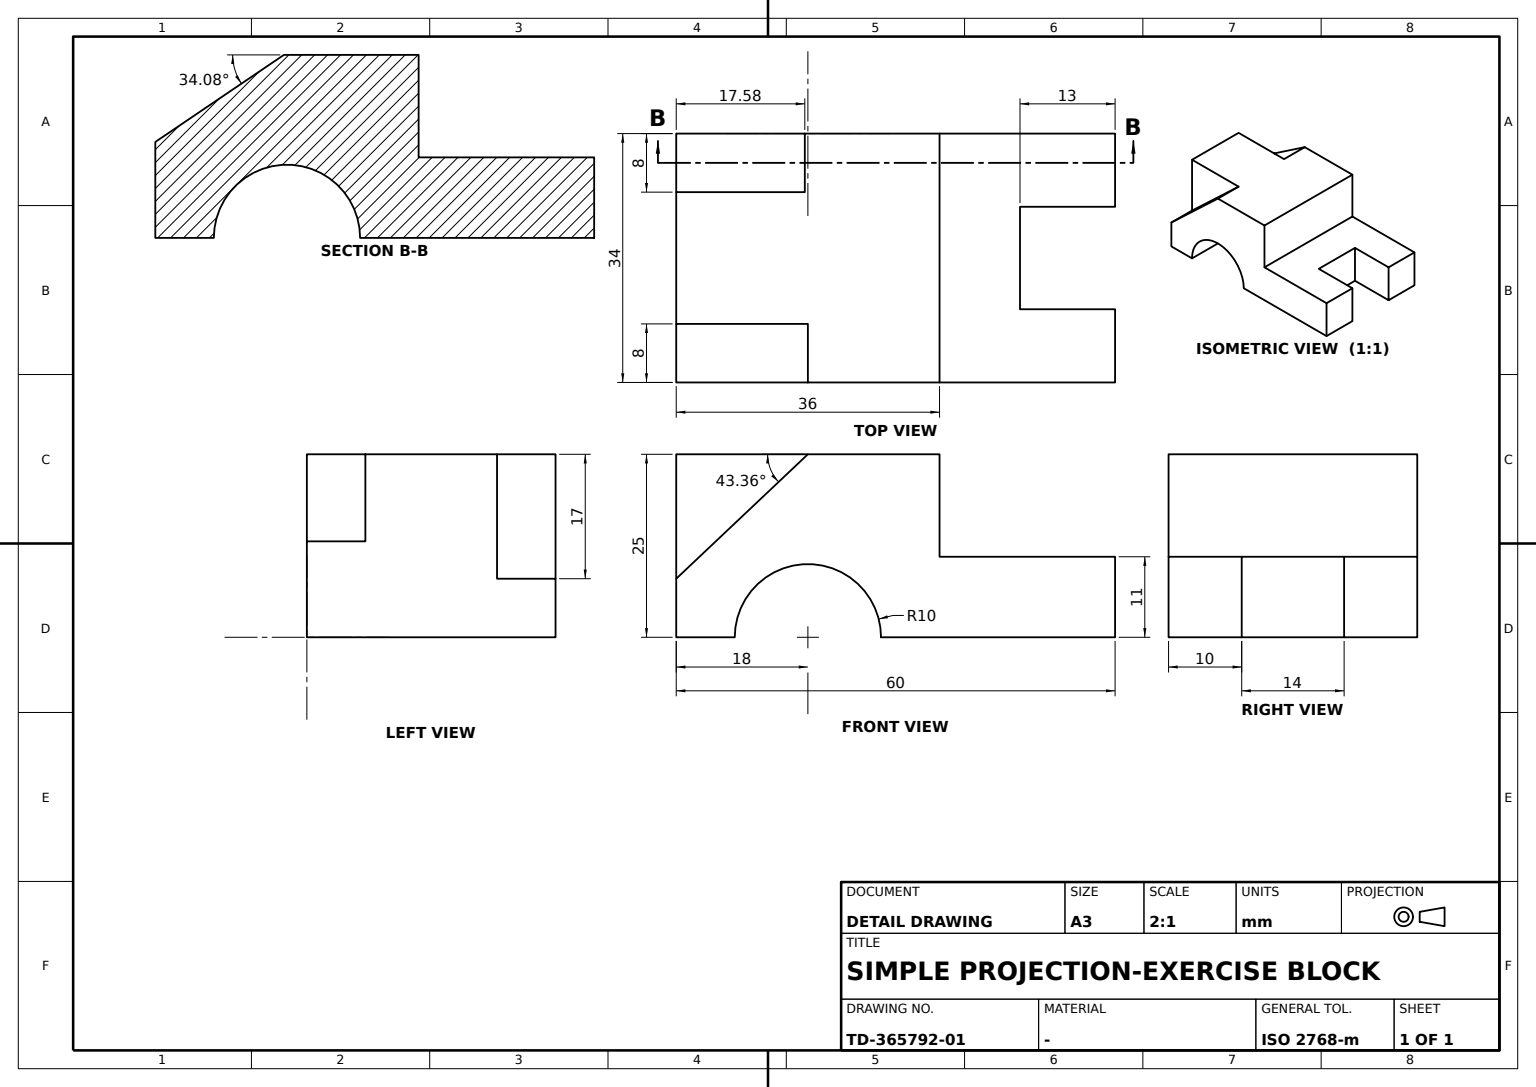
ISO-10303-21;
HEADER;
FILE_DESCRIPTION((''),'2;1');
FILE_NAME('','',(''),(''),'','','');
FILE_SCHEMA(('AUTOMOTIVE_DESIGN'));
ENDSEC;
DATA;
#1=APPLICATION_CONTEXT('');
#2=PRODUCT_CONTEXT('',#1,'mechanical');
#3=PRODUCT('','','',(#2));
#4=PRODUCT_DEFINITION_FORMATION('','',#3);
#5=PRODUCT_DEFINITION_CONTEXT('',#1,'design');
#6=PRODUCT_DEFINITION('','',#4,#5);
#7=PRODUCT_DEFINITION_SHAPE('','',#6);
#8=(LENGTH_UNIT()NAMED_UNIT(*)SI_UNIT(.MILLI.,.METRE.));
#9=(NAMED_UNIT(*)PLANE_ANGLE_UNIT()SI_UNIT($,.RADIAN.));
#10=(NAMED_UNIT(*)SI_UNIT($,.STERADIAN.)SOLID_ANGLE_UNIT());
#11=UNCERTAINTY_MEASURE_WITH_UNIT(LENGTH_MEASURE(0.005),#8,'distance_accuracy_value','');
#12=(GEOMETRIC_REPRESENTATION_CONTEXT(3)GLOBAL_UNCERTAINTY_ASSIGNED_CONTEXT((#11))GLOBAL_UNIT_ASSIGNED_CONTEXT((#8,#9,#10))REPRESENTATION_CONTEXT('',''));
#13=CARTESIAN_POINT('',(-17.,-18.,13.105238));
#14=VERTEX_POINT('',#13);
#15=CARTESIAN_POINT('',(-9.,-18.,13.105238));
#16=VERTEX_POINT('',#15);
#17=DIRECTION('',(1.,0.,0.));
#18=VECTOR('',#17,1000.);
#19=LINE('',#13,#18);
#20=EDGE_CURVE('',#14,#16,#19,.T.);
#21=ORIENTED_EDGE('',*,*,#20,.T.);
#22=CARTESIAN_POINT('',(-9.,-0.420078,25.));
#23=VERTEX_POINT('',#22);
#24=DIRECTION('',(0.,-0.82822958,-0.560388939));
#25=VECTOR('',#24,1000.);
#26=LINE('',#22,#25);
#27=EDGE_CURVE('',#23,#16,#26,.T.);
#28=ORIENTED_EDGE('',*,*,#27,.F.);
#29=CARTESIAN_POINT('',(-17.,-0.420078,25.));
#30=VERTEX_POINT('',#29);
#31=CARTESIAN_POINT('',(0.,-0.420078,25.));
#32=LINE('',#31,#18);
#33=EDGE_CURVE('',#30,#23,#32,.T.);
#34=ORIENTED_EDGE('',*,*,#33,.F.);
#35=CARTESIAN_POINT('',(-17.,-11.735187,17.344077));
#36=LINE('',#35,#25);
#37=EDGE_CURVE('',#30,#14,#36,.T.);
#38=ORIENTED_EDGE('',*,*,#37,.T.);
#39=EDGE_LOOP('',(#21,#28,#34,#38));
#40=FACE_BOUND('',#39,.T.);
#41=DIRECTION('',(0.,-0.560388939,0.82822958));
#42=AXIS2_PLACEMENT_3D('',#29,#41,#24);
#43=PLANE('',#42);
#44=ADVANCED_FACE('',(#40),#43,.T.);
#45=CARTESIAN_POINT('',(-17.,42.,11.));
#46=VERTEX_POINT('',#45);
#47=CARTESIAN_POINT('',(-7.,42.,11.));
#48=VERTEX_POINT('',#47);
#49=CARTESIAN_POINT('',(0.,42.,11.));
#50=LINE('',#49,#18);
#51=EDGE_CURVE('',#46,#48,#50,.T.);
#52=ORIENTED_EDGE('',*,*,#51,.F.);
#53=CARTESIAN_POINT('',(-17.,18.,11.));
#54=VERTEX_POINT('',#53);
#55=CARTESIAN_POINT('',(-17.,0.,11.));
#56=DIRECTION('',(0.,-1.,0.));
#57=VECTOR('',#56,1000.);
#58=LINE('',#55,#57);
#59=EDGE_CURVE('',#46,#54,#58,.T.);
#60=ORIENTED_EDGE('',*,*,#59,.T.);
#61=CARTESIAN_POINT('',(17.,18.,11.));
#62=VERTEX_POINT('',#61);
#63=CARTESIAN_POINT('',(0.,18.,11.));
#64=LINE('',#63,#18);
#65=EDGE_CURVE('',#54,#62,#64,.T.);
#66=ORIENTED_EDGE('',*,*,#65,.T.);
#67=CARTESIAN_POINT('',(17.,42.,11.));
#68=VERTEX_POINT('',#67);
#69=CARTESIAN_POINT('',(17.,0.,11.));
#70=LINE('',#69,#57);
#71=EDGE_CURVE('',#68,#62,#70,.T.);
#72=ORIENTED_EDGE('',*,*,#71,.F.);
#73=CARTESIAN_POINT('',(7.,42.,11.));
#74=VERTEX_POINT('',#73);
#75=EDGE_CURVE('',#74,#68,#50,.T.);
#76=ORIENTED_EDGE('',*,*,#75,.F.);
#77=CARTESIAN_POINT('',(7.,29.,11.));
#78=VERTEX_POINT('',#77);
#79=LINE('',#73,#57);
#80=EDGE_CURVE('',#74,#78,#79,.T.);
#81=ORIENTED_EDGE('',*,*,#80,.T.);
#82=CARTESIAN_POINT('',(-7.,29.,11.));
#83=VERTEX_POINT('',#82);
#84=DIRECTION('',(-1.,0.,0.));
#85=VECTOR('',#84,1000.);
#86=LINE('',#77,#85);
#87=EDGE_CURVE('',#78,#83,#86,.T.);
#88=ORIENTED_EDGE('',*,*,#87,.T.);
#89=DIRECTION('',(0.,1.,0.));
#90=VECTOR('',#89,1000.);
#91=LINE('',#82,#90);
#92=EDGE_CURVE('',#83,#48,#91,.T.);
#93=ORIENTED_EDGE('',*,*,#92,.T.);
#94=EDGE_LOOP('',(#52,#60,#66,#72,#76,#81,#88,#93));
#95=FACE_BOUND('',#94,.T.);
#96=DIRECTION('',(0.,0.,1.));
#97=AXIS2_PLACEMENT_3D('',#49,#96,#56);
#98=PLANE('',#97);
#99=ADVANCED_FACE('',(#95),#98,.T.);
#100=ORIENTED_EDGE('',*,*,#33,.T.);
#101=CARTESIAN_POINT('',(-9.,-18.,25.));
#102=VERTEX_POINT('',#101);
#103=CARTESIAN_POINT('',(-9.,18.,25.));
#104=LINE('',#103,#57);
#105=EDGE_CURVE('',#23,#102,#104,.T.);
#106=ORIENTED_EDGE('',*,*,#105,.T.);
#107=CARTESIAN_POINT('',(9.,-18.,25.));
#108=VERTEX_POINT('',#107);
#109=CARTESIAN_POINT('',(0.,-18.,25.));
#110=LINE('',#109,#18);
#111=EDGE_CURVE('',#102,#108,#110,.T.);
#112=ORIENTED_EDGE('',*,*,#111,.T.);
#113=CARTESIAN_POINT('',(9.,0.,25.));
#114=VERTEX_POINT('',#113);
#115=LINE('',#113,#57);
#116=EDGE_CURVE('',#114,#108,#115,.T.);
#117=ORIENTED_EDGE('',*,*,#116,.F.);
#118=CARTESIAN_POINT('',(17.,0.,25.));
#119=VERTEX_POINT('',#118);
#120=LINE('',#118,#85);
#121=EDGE_CURVE('',#119,#114,#120,.T.);
#122=ORIENTED_EDGE('',*,*,#121,.F.);
#123=CARTESIAN_POINT('',(17.,18.,25.));
#124=VERTEX_POINT('',#123);
#125=LINE('',#118,#57);
#126=EDGE_CURVE('',#124,#119,#125,.T.);
#127=ORIENTED_EDGE('',*,*,#126,.F.);
#128=CARTESIAN_POINT('',(-17.,18.,25.));
#129=VERTEX_POINT('',#128);
#130=CARTESIAN_POINT('',(0.,18.,25.));
#131=LINE('',#130,#18);
#132=EDGE_CURVE('',#129,#124,#131,.T.);
#133=ORIENTED_EDGE('',*,*,#132,.F.);
#134=CARTESIAN_POINT('',(-17.,0.,25.));
#135=LINE('',#134,#57);
#136=EDGE_CURVE('',#129,#30,#135,.T.);
#137=ORIENTED_EDGE('',*,*,#136,.T.);
#138=EDGE_LOOP('',(#100,#106,#112,#117,#122,#127,#133,#137));
#139=FACE_BOUND('',#138,.T.);
#140=AXIS2_PLACEMENT_3D('',#130,#96,#56);
#141=PLANE('',#140);
#142=ADVANCED_FACE('',(#139),#141,.T.);
#143=CARTESIAN_POINT('',(17.,-18.,0.));
#144=VERTEX_POINT('',#143);
#145=CARTESIAN_POINT('',(17.,-10.,0.));
#146=VERTEX_POINT('',#145);
#147=CARTESIAN_POINT('',(17.,0.,0.));
#148=LINE('',#147,#90);
#149=EDGE_CURVE('',#144,#146,#148,.T.);
#150=ORIENTED_EDGE('',*,*,#149,.F.);
#151=CARTESIAN_POINT('',(-17.,-18.,0.));
#152=VERTEX_POINT('',#151);
#153=CARTESIAN_POINT('',(0.,-18.,0.));
#154=LINE('',#153,#18);
#155=EDGE_CURVE('',#152,#144,#154,.T.);
#156=ORIENTED_EDGE('',*,*,#155,.F.);
#157=CARTESIAN_POINT('',(-17.,-10.,0.));
#158=VERTEX_POINT('',#157);
#159=CARTESIAN_POINT('',(-17.,0.,0.));
#160=LINE('',#159,#90);
#161=EDGE_CURVE('',#152,#158,#160,.T.);
#162=ORIENTED_EDGE('',*,*,#161,.T.);
#163=LINE('',#157,#18);
#164=EDGE_CURVE('',#158,#146,#163,.T.);
#165=ORIENTED_EDGE('',*,*,#164,.T.);
#166=EDGE_LOOP('',(#150,#156,#162,#165));
#167=FACE_BOUND('',#166,.T.);
#168=DIRECTION('',(0.,0.,-1.));
#169=AXIS2_PLACEMENT_3D('',#153,#168,#89);
#170=PLANE('',#169);
#171=ADVANCED_FACE('',(#167),#170,.T.);
#172=CARTESIAN_POINT('',(7.,29.,0.));
#173=VERTEX_POINT('',#172);
#174=VECTOR('',#168,1000.);
#175=LINE('',#77,#174);
#176=EDGE_CURVE('',#78,#173,#175,.T.);
#177=ORIENTED_EDGE('',*,*,#176,.F.);
#178=ORIENTED_EDGE('',*,*,#80,.F.);
#179=CARTESIAN_POINT('',(7.,42.,0.));
#180=VERTEX_POINT('',#179);
#181=LINE('',#179,#174);
#182=EDGE_CURVE('',#74,#180,#181,.T.);
#183=ORIENTED_EDGE('',*,*,#182,.T.);
#184=CARTESIAN_POINT('',(7.,-18.,0.));
#185=LINE('',#184,#57);
#186=EDGE_CURVE('',#180,#173,#185,.T.);
#187=ORIENTED_EDGE('',*,*,#186,.T.);
#188=EDGE_LOOP('',(#177,#178,#183,#187));
#189=FACE_BOUND('',#188,.T.);
#190=AXIS2_PLACEMENT_3D('',#73,#17,#56);
#191=PLANE('',#190);
#192=ADVANCED_FACE('',(#189),#191,.F.);
#193=CARTESIAN_POINT('',(17.,-18.,8.));
#194=VERTEX_POINT('',#193);
#195=DIRECTION('',(0.,0.727013153,0.686623533));
#196=VECTOR('',#195,1000.);
#197=LINE('',#193,#196);
#198=EDGE_CURVE('',#194,#119,#197,.T.);
#199=ORIENTED_EDGE('',*,*,#198,.T.);
#200=ORIENTED_EDGE('',*,*,#121,.T.);
#201=CARTESIAN_POINT('',(9.,-18.,8.));
#202=VERTEX_POINT('',#201);
#203=LINE('',#201,#196);
#204=EDGE_CURVE('',#202,#114,#203,.T.);
#205=ORIENTED_EDGE('',*,*,#204,.F.);
#206=CARTESIAN_POINT('',(0.,-18.,8.));
#207=LINE('',#206,#85);
#208=EDGE_CURVE('',#194,#202,#207,.T.);
#209=ORIENTED_EDGE('',*,*,#208,.F.);
#210=EDGE_LOOP('',(#199,#200,#205,#209));
#211=FACE_BOUND('',#210,.T.);
#212=DIRECTION('',(0.,-0.686623533,0.727013153));
#213=AXIS2_PLACEMENT_3D('',#193,#212,#195);
#214=PLANE('',#213);
#215=ADVANCED_FACE('',(#211),#214,.T.);
#216=LINE('',#101,#174);
#217=EDGE_CURVE('',#102,#16,#216,.T.);
#218=ORIENTED_EDGE('',*,*,#217,.F.);
#219=ORIENTED_EDGE('',*,*,#105,.F.);
#220=ORIENTED_EDGE('',*,*,#27,.T.);
#221=EDGE_LOOP('',(#218,#219,#220));
#222=FACE_BOUND('',#221,.T.);
#223=CARTESIAN_POINT('',(-9.,0.,0.));
#224=AXIS2_PLACEMENT_3D('',#223,#84,#56);
#225=PLANE('',#224);
#226=ADVANCED_FACE('',(#222),#225,.T.);
#227=ORIENTED_EDGE('',*,*,#186,.F.);
#228=CARTESIAN_POINT('',(17.,42.,0.));
#229=VERTEX_POINT('',#228);
#230=CARTESIAN_POINT('',(0.,42.,0.));
#231=LINE('',#230,#18);
#232=EDGE_CURVE('',#180,#229,#231,.T.);
#233=ORIENTED_EDGE('',*,*,#232,.T.);
#234=CARTESIAN_POINT('',(17.,10.,0.));
#235=VERTEX_POINT('',#234);
#236=EDGE_CURVE('',#235,#229,#148,.T.);
#237=ORIENTED_EDGE('',*,*,#236,.F.);
#238=CARTESIAN_POINT('',(-17.,10.,0.));
#239=VERTEX_POINT('',#238);
#240=LINE('',#238,#18);
#241=EDGE_CURVE('',#239,#235,#240,.T.);
#242=ORIENTED_EDGE('',*,*,#241,.F.);
#243=CARTESIAN_POINT('',(-17.,42.,0.));
#244=VERTEX_POINT('',#243);
#245=EDGE_CURVE('',#239,#244,#160,.T.);
#246=ORIENTED_EDGE('',*,*,#245,.T.);
#247=CARTESIAN_POINT('',(-7.,42.,0.));
#248=VERTEX_POINT('',#247);
#249=EDGE_CURVE('',#244,#248,#231,.T.);
#250=ORIENTED_EDGE('',*,*,#249,.T.);
#251=CARTESIAN_POINT('',(-7.,29.,0.));
#252=VERTEX_POINT('',#251);
#253=LINE('',#251,#57);
#254=EDGE_CURVE('',#248,#252,#253,.T.);
#255=ORIENTED_EDGE('',*,*,#254,.T.);
#256=CARTESIAN_POINT('',(0.,29.,0.));
#257=LINE('',#256,#85);
#258=EDGE_CURVE('',#173,#252,#257,.T.);
#259=ORIENTED_EDGE('',*,*,#258,.F.);
#260=EDGE_LOOP('',(#227,#233,#237,#242,#246,#250,#255,#259));
#261=FACE_BOUND('',#260,.T.);
#262=ADVANCED_FACE('',(#261),#170,.T.);
#263=CARTESIAN_POINT('',(9.,-18.,0.));
#264=LINE('',#263,#174);
#265=EDGE_CURVE('',#108,#202,#264,.T.);
#266=ORIENTED_EDGE('',*,*,#265,.T.);
#267=ORIENTED_EDGE('',*,*,#204,.T.);
#268=ORIENTED_EDGE('',*,*,#116,.T.);
#269=EDGE_LOOP('',(#266,#267,#268));
#270=FACE_BOUND('',#269,.T.);
#271=CARTESIAN_POINT('',(9.,0.,0.));
#272=AXIS2_PLACEMENT_3D('',#271,#17,#89);
#273=PLANE('',#272);
#274=ADVANCED_FACE('',(#270),#273,.T.);
#275=AXIS2_PLACEMENT_3D('',#147,#17,#168);
#276=CIRCLE('',#275,10.);
#277=EDGE_CURVE('',#235,#146,#276,.T.);
#278=ORIENTED_EDGE('',*,*,#277,.T.);
#279=ORIENTED_EDGE('',*,*,#164,.F.);
#280=AXIS2_PLACEMENT_3D('',#159,#17,#168);
#281=CIRCLE('',#280,10.);
#282=EDGE_CURVE('',#239,#158,#281,.T.);
#283=ORIENTED_EDGE('',*,*,#282,.F.);
#284=ORIENTED_EDGE('',*,*,#241,.T.);
#285=EDGE_LOOP('',(#278,#279,#283,#284));
#286=FACE_BOUND('',#285,.T.);
#287=CARTESIAN_POINT('',(0.,0.,0.));
#288=AXIS2_PLACEMENT_3D('',#287,#17,#89);
#289=CYLINDRICAL_SURFACE('',#288,10.);
#290=ADVANCED_FACE('',(#286),#289,.F.);
#291=ORIENTED_EDGE('',*,*,#65,.F.);
#292=CARTESIAN_POINT('',(-17.,18.,0.));
#293=VECTOR('',#96,1000.);
#294=LINE('',#292,#293);
#295=EDGE_CURVE('',#54,#129,#294,.T.);
#296=ORIENTED_EDGE('',*,*,#295,.T.);
#297=ORIENTED_EDGE('',*,*,#132,.T.);
#298=CARTESIAN_POINT('',(17.,18.,0.));
#299=LINE('',#298,#293);
#300=EDGE_CURVE('',#62,#124,#299,.T.);
#301=ORIENTED_EDGE('',*,*,#300,.F.);
#302=EDGE_LOOP('',(#291,#296,#297,#301));
#303=FACE_BOUND('',#302,.T.);
#304=AXIS2_PLACEMENT_3D('',#63,#89,#96);
#305=PLANE('',#304);
#306=ADVANCED_FACE('',(#303),#305,.T.);
#307=ORIENTED_EDGE('',*,*,#136,.F.);
#308=ORIENTED_EDGE('',*,*,#295,.F.);
#309=ORIENTED_EDGE('',*,*,#59,.F.);
#310=LINE('',#243,#293);
#311=EDGE_CURVE('',#244,#46,#310,.T.);
#312=ORIENTED_EDGE('',*,*,#311,.F.);
#313=ORIENTED_EDGE('',*,*,#245,.F.);
#314=ORIENTED_EDGE('',*,*,#282,.T.);
#315=ORIENTED_EDGE('',*,*,#161,.F.);
#316=LINE('',#151,#174);
#317=EDGE_CURVE('',#14,#152,#316,.T.);
#318=ORIENTED_EDGE('',*,*,#317,.F.);
#319=ORIENTED_EDGE('',*,*,#37,.F.);
#320=EDGE_LOOP('',(#307,#308,#309,#312,#313,#314,#315,#318,#319));
#321=FACE_BOUND('',#320,.T.);
#322=AXIS2_PLACEMENT_3D('',#159,#17,#89);
#323=PLANE('',#322);
#324=ADVANCED_FACE('',(#321),#323,.F.);
#325=LINE('',#82,#174);
#326=EDGE_CURVE('',#83,#252,#325,.T.);
#327=ORIENTED_EDGE('',*,*,#326,.F.);
#328=ORIENTED_EDGE('',*,*,#87,.F.);
#329=ORIENTED_EDGE('',*,*,#176,.T.);
#330=ORIENTED_EDGE('',*,*,#258,.T.);
#331=EDGE_LOOP('',(#327,#328,#329,#330));
#332=FACE_BOUND('',#331,.T.);
#333=AXIS2_PLACEMENT_3D('',#77,#56,#84);
#334=PLANE('',#333);
#335=ADVANCED_FACE('',(#332),#334,.F.);
#336=LINE('',#47,#174);
#337=EDGE_CURVE('',#48,#248,#336,.T.);
#338=ORIENTED_EDGE('',*,*,#337,.F.);
#339=ORIENTED_EDGE('',*,*,#92,.F.);
#340=ORIENTED_EDGE('',*,*,#326,.T.);
#341=ORIENTED_EDGE('',*,*,#254,.F.);
#342=EDGE_LOOP('',(#338,#339,#340,#341));
#343=FACE_BOUND('',#342,.T.);
#344=AXIS2_PLACEMENT_3D('',#82,#84,#89);
#345=PLANE('',#344);
#346=ADVANCED_FACE('',(#343),#345,.F.);
#347=ORIENTED_EDGE('',*,*,#249,.F.);
#348=ORIENTED_EDGE('',*,*,#311,.T.);
#349=ORIENTED_EDGE('',*,*,#51,.T.);
#350=ORIENTED_EDGE('',*,*,#337,.T.);
#351=EDGE_LOOP('',(#347,#348,#349,#350));
#352=FACE_BOUND('',#351,.T.);
#353=AXIS2_PLACEMENT_3D('',#230,#89,#96);
#354=PLANE('',#353);
#355=ADVANCED_FACE('',(#352),#354,.T.);
#356=ORIENTED_EDGE('',*,*,#20,.F.);
#357=ORIENTED_EDGE('',*,*,#317,.T.);
#358=ORIENTED_EDGE('',*,*,#155,.T.);
#359=LINE('',#143,#174);
#360=EDGE_CURVE('',#194,#144,#359,.T.);
#361=ORIENTED_EDGE('',*,*,#360,.F.);
#362=ORIENTED_EDGE('',*,*,#208,.T.);
#363=ORIENTED_EDGE('',*,*,#265,.F.);
#364=ORIENTED_EDGE('',*,*,#111,.F.);
#365=ORIENTED_EDGE('',*,*,#217,.T.);
#366=EDGE_LOOP('',(#356,#357,#358,#361,#362,#363,#364,#365));
#367=FACE_BOUND('',#366,.T.);
#368=AXIS2_PLACEMENT_3D('',#109,#56,#168);
#369=PLANE('',#368);
#370=ADVANCED_FACE('',(#367),#369,.T.);
#371=ORIENTED_EDGE('',*,*,#75,.T.);
#372=LINE('',#228,#293);
#373=EDGE_CURVE('',#229,#68,#372,.T.);
#374=ORIENTED_EDGE('',*,*,#373,.F.);
#375=ORIENTED_EDGE('',*,*,#232,.F.);
#376=ORIENTED_EDGE('',*,*,#182,.F.);
#377=EDGE_LOOP('',(#371,#374,#375,#376));
#378=FACE_BOUND('',#377,.T.);
#379=ADVANCED_FACE('',(#378),#354,.T.);
#380=ORIENTED_EDGE('',*,*,#236,.T.);
#381=ORIENTED_EDGE('',*,*,#373,.T.);
#382=ORIENTED_EDGE('',*,*,#71,.T.);
#383=ORIENTED_EDGE('',*,*,#300,.T.);
#384=ORIENTED_EDGE('',*,*,#126,.T.);
#385=ORIENTED_EDGE('',*,*,#198,.F.);
#386=ORIENTED_EDGE('',*,*,#360,.T.);
#387=ORIENTED_EDGE('',*,*,#149,.T.);
#388=ORIENTED_EDGE('',*,*,#277,.F.);
#389=EDGE_LOOP('',(#380,#381,#382,#383,#384,#385,#386,#387,#388));
#390=FACE_BOUND('',#389,.T.);
#391=AXIS2_PLACEMENT_3D('',#147,#17,#89);
#392=PLANE('',#391);
#393=ADVANCED_FACE('',(#390),#392,.T.);
#394=CLOSED_SHELL('',(#44,#99,#142,#171,#192,#215,#226,#262,#274,#290,#306,#324,#335,#346,#355,#370,#379,#393));
#395=MANIFOLD_SOLID_BREP('',#394);
#396=ADVANCED_BREP_SHAPE_REPRESENTATION('',(#395),#12);
#397=SHAPE_DEFINITION_REPRESENTATION(#7,#396);
ENDSEC;
END-ISO-10303-21;
